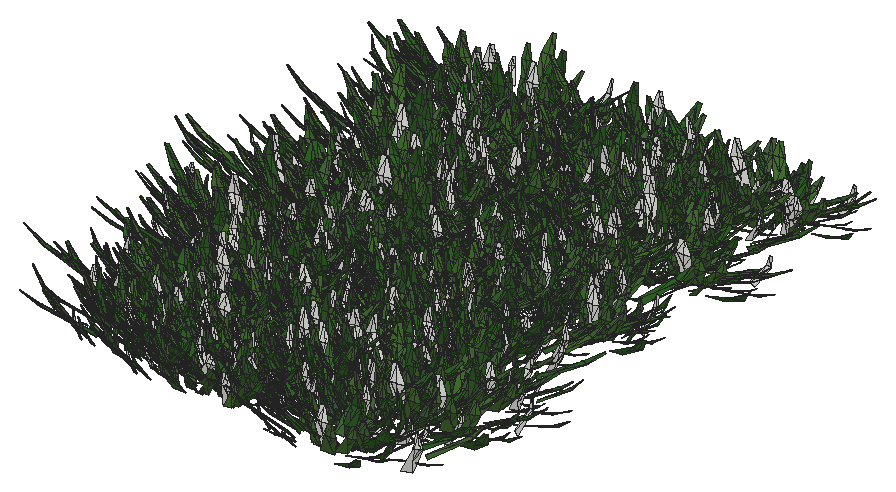
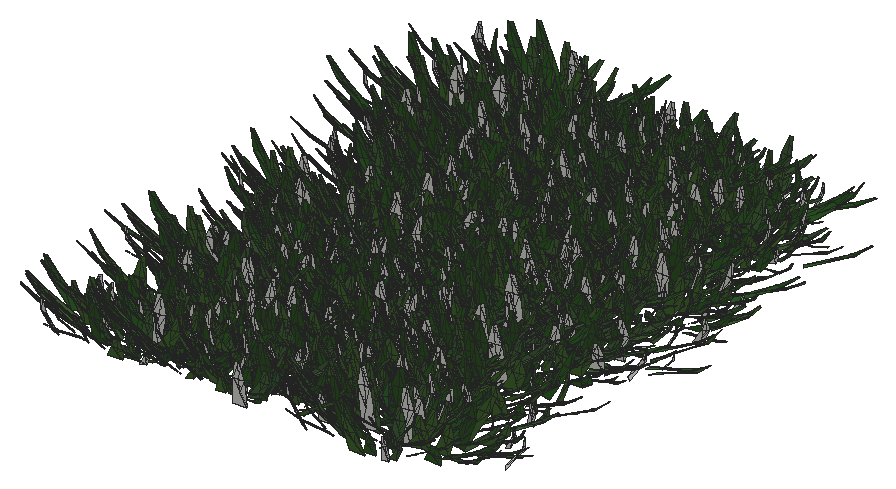
# SketchUp Ruby script. Lengths in inches.
U = 1.inch
M = Sketchup.active_model
def pt(a) = Geom::Point3d.new(a.map { |v| v * U })
def face(e, loops, mat)
  f = e.add_face(loops[0].map { |a| pt(a) })
  loops[1..].each { |l| e.add_face(l.map { |a| pt(a) }).erase! }
  f.material = f.back_material = mat if mat
  f
end
# faces: each face lists its corners as indices into pts; further lists are holes
def faces(e, pts, list, mat = nil) = list.each { |f| face(e, (f[0].is_a?(Array) ? f : [f]).map { |l| l.map { |i| pts[i] } }, mat) }
# xy, xz, yz: faces in a plane at the given z, y or x. An outline is a flat list of corners, or four numbers for a rectangle; further outlines are holes
def ring(l) = l.size == 4 ? [[l[0], l[1]], [l[2], l[1]], [l[2], l[3]], [l[0], l[3]]] : l.each_slice(2).to_a
def flat(e, list, mat, &to3) = list.each { |f| face(e, (f[0].is_a?(Array) ? f : [f]).map { |l| ring(l).map { |u, v| to3.(u, v) } }, mat) }
def xy(e, z, list, mat = nil) = flat(e, list, mat) { |x, y| [x, y, z] }
def xz(e, y, list, mat = nil) = flat(e, list, mat) { |x, z| [x, y, z] }
def yz(e, x, list, mat = nil) = flat(e, list, mat) { |y, z| [x, y, z] }
def lines(e, pts, list) = list.each { |a, b| e.add_line(pt(pts[a]), pt(pts[b])) }
# prism: a flat outline (further loops are holes) pulled along v
def prism(e, loops, v, mat = nil)
  f = face(e, loops, mat); d = Geom::Vector3d.new(v.map { |x| x * U })
  f.pushpull(f.normal.samedirection?(d) ? d.length : -d.length)
end
def box(e, o, s, mat = nil) = prism(e, [[o, [o[0] + s[0], o[1], o[2]], [o[0] + s[0], o[1] + s[1], o[2]], [o[0], o[1] + s[1], o[2]]]], [0, 0, s[2]], mat)
def at(x, y, z, deg = 0) = Geom::Transformation.translation(pt([x, y, z])) * Geom::Transformation.rotation(ORIGIN, Z_AXIS, deg.degrees)
def axes(o, x, y, z) = Geom::Transformation.new([*x, 0, *y, 0, *z, 0, *pt(o).to_a, 1])
def part(name) = M.definitions.add(name)
# library, detail: a bought-in or finely detailed component or shape, given as its bounding box
def library(name, o, s) = part(name).tap { |d| box(d.entities, o, s) }
def detail(e, o, s) = box(e.add_group.entities, o, s)
def put(e, d, t, mat = nil) = e.add_instance(d, t).tap { |i| i.material = mat if mat }
def group(e, t, mat = nil) = e.add_group.tap { |g| g.transformation = t; g.material = mat if mat }.entities
root = M.entities
M.materials.add("Material82").color = [68, 110, 58]
M.materials.add("Material83").color = [48, 90, 38]
M.materials.add("Material84").color = [68, 110, 48]
M.materials.add("Material85").color = [48, 90, 48]
M.materials.add("Material86").color = [58, 110, 58]
M.materials.add("Material87").color = [58, 90, 38]
M.materials.add("Material88").color = [68, 100, 58]
M.materials.add("Material89").color = [48, 100, 38]
c1 = part("grass00")
p = [[-0.6875,0.15,0],[-0.56,0.08,5.52],[-0.04,0.03,2.76],[0.48,-0.02,0],[0.35,-0.02,5.52],[-0.1,-0.14,5.52],
  [-0.12,0.65,8.37],[-0.42,0.65,8.37]]
faces(c1.entities,p,[[0,1,2,3],[3,2,4],[1,5,2],[5,4,2],[1,6,5],[4,5,6],[7,6,1]])
c2 = part("Group16\#1")
put(c2.entities,c1,axes([1.44,-0.61,-0.01],[0.05352,0.12609,0],[-0.10704,0.04543,0.07239],[0.06664,-0.02828,0.11628]),"Material85")
put(c2.entities,c1,axes([0.76,-0.15,-0.01],[0.04676,0.24062,0],[-0.23162,0.04501,0.06642],[0.0652,-0.01267,0.23595]),"Material82")
put(c2.entities,c1,axes([0.79,0.01,-0.01],[-0.00606,0.34651,0],[-0.34381,-0.00602,0.0432],[0.04319,0.00076,0.34386]))
put(c2.entities,c1,axes([1,0.23,-0.01],[-0.07192,0.31144,0],[-0.28722,-0.06632,0.1236],[0.12043,0.02781,0.29478]),"Material84")
put(c2.entities,c1,axes([1.66,0.77,-0.01],[-0.13828,0.29651,0],[-0.21551,-0.1005,0.22471],[0.20365,0.09498,0.23779]),"Material89")
put(c2.entities,c1,axes([0.6875,0.52,-0.01],[-0.18126,0.24051,0],[-0.22746,-0.17142,0.09788],[0.07817,0.05891,0.28481]),"Material84")
put(c2.entities,c1,axes([0.68,0.78,-0.01],[-0.215,0.18688,0],[-0.12385,-0.14248,0.21334],[0.13995,0.16101,0.18878]),"Material82")
put(c2.entities,c1,axes([0.56,1,-0.01],[-0.13756,0.07624,0],[-0.06159,-0.11112,0.0927],[0.04494,0.08108,0.12705]),"Material84")
put(c2.entities,c1,axes([0.2,0.64,-0.01],[-0.23729,0.07254,0],[-0.05711,-0.18681,0.153],[0.04473,0.14632,0.19535]),"Material89")
put(c2.entities,c1,axes([0.0625,0.72,-0.01],[-0.28874,0.02525,0],[-0.02179,-0.24916,0.14647],[0.01276,0.14591,0.25012]),"Material82")
put(c2.entities,c1,axes([-0.08,0.62,-0.01],[-0.34089,-0.04187,0],[0.03255,-0.26504,0.216],[-0.02633,0.21439,0.26703]),"Material89")
put(c2.entities,c1,axes([-0.34,0.98,-0.01],[-0.14314,-0.0493,0],[0.04397,-0.12769,0.06843],[-0.02228,0.0647,0.13505]),"Material89")
put(c2.entities,c1,axes([-0.87,1.45,-0.01],[-0.23488,-0.14114,0],[0.13761,-0.22901,0.06087],[-0.03135,0.05217,0.26717]))
put(c2.entities,c1,axes([-0.72,0.77,-0.01],[-0.14208,-0.13251,0],[0.07209,-0.0773,0.16301],[-0.11118,0.11922,0.1057]),"Material89")
put(c2.entities,c1,axes([-0.62,0.43,-0.01],[-0.14845,-0.21203,0],[0.18654,-0.13061,0.12304],[-0.10079,0.07057,0.22772]),"Material82")
put(c2.entities,c1,axes([-0.68,0.29,-0.01],[-0.13639,-0.32136,0],[0.31723,-0.13464,0.05579],[-0.05136,0.0218,0.34462]),"Material83")
put(c2.entities,c1,axes([-0.64,0.125,-0.01],[-0.0458,-0.23569,0],[0.22124,-0.043,0.08276],[-0.08124,0.01579,0.22538]),"Material86")
put(c2.entities,c1,axes([-1.6,-0.03,-0.01],[0.00576,-0.32897,0],[0.27526,0.00482,0.18018],[-0.18015,-0.00315,0.2753]),"Material84")
put(c2.entities,c1,axes([-1.36,-0.31,-0.01],[0.05718,-0.24765,0],[0.18172,0.04196,0.17267],[-0.16825,-0.03885,0.1865]),"Material89")
put(c2.entities,c1,axes([-1.54,-0.72,-0.01],[0.06537,-0.14017,0],[0.13555,0.06321,0.03939],[-0.0357,-0.01665,0.14956]))
put(c2.entities,c1,axes([-1.19,-0.9,-0.01],[0.09597,-0.12735,0],[0.11214,0.08451,0.07557],[-0.06035,-0.04548,0.14042]),"Material88")
put(c2.entities,c1,axes([-0.47,-0.54,-0.01],[0.11588,-0.10072,0],[0.0618,0.0711,0.12124],[-0.07953,-0.0915,0.0942]))
put(c2.entities,c1,axes([-0.47,-0.84,-0.01],[0.11927,-0.0661,0],[0.06603,0.11913,0.00646],[-0.00313,-0.00565,0.13621]),"Material84")
put(c2.entities,c1,axes([-0.38,-1.24,-0.01],[0.28037,-0.08571,0],[0.0618,0.20215,0.20315],[-0.05939,-0.19428,0.21139]),"Material88")
put(c2.entities,c1,axes([-0.06,-0.66,-0.01],[0.22719,-0.01987,0],[0.01247,0.14255,0.17758],[-0.01547,-0.17691,0.1431]),"Material87")
put(c2.entities,c1,axes([0.11,-0.89,-0.01],[0.14882,0.01828,0],[-0.01058,0.08611,0.12229],[0.01491,-0.12138,0.08676]),"Material85")
put(c2.entities,c1,axes([0.25,-0.72,-0.01],[0.20481,0.07053,0],[-0.06206,0.18022,0.10291],[0.03351,-0.0973,0.1906]),"Material85")
put(c2.entities,c1,axes([0.85,-1.42,-0.01],[0.16481,0.09904,0],[-0.09472,0.15762,0.05616],[0.02893,-0.04814,0.18389]),"Material84")
put(c2.entities,c1,axes([1.01,-1.09,-0.01],[0.21858,0.20385,0],[-0.17495,0.1876,0.15339],[0.10462,-0.11218,0.25652]),"Material89")
put(c2.entities,c1,axes([1.01,-0.71,-0.01],[0.08733,0.12473,0],[-0.06445,0.04512,0.13037],[0.1068,-0.07477,0.07867]),"Material85")
c3 = part("Group15\#1")
put(c3.entities,c2,at(0,0,0))
c4 = part("3darcstudiotree_grass00\#1")
put(c4.entities,c3,at(0,0,0))
put(root,c4,axes([650.38,940.35,-29.74],[0.55958,-1.81201,0],[3.80263,0.18264,-0.0324],[0.16574,0.00796,1.47946]))
put(root,c4,axes([635.88,940.68,-29.74],[3.74746,0.48768,0],[-1.05117,1.25627,-0.0401],[-0.08448,0.10096,1.69032]))
put(root,c4,axes([652.35,941.68,-29.74],[-3.98203,-0.87024,0],[2.1917,-1.55976,-0.02403],[0.066,-0.04697,1.92026]))
put(root,c4,axes([638.66,941.92,-29.74],[-3.4101,0.33219,0],[-0.86784,-1.38556,-0.03348],[-0.045,-0.07185,1.52035]))
put(root,c4,axes([627.54,942.55,-29.74],[3.16343,0.45899,0],[-1.51538,1.62437,-0.05896],[-0.12026,0.12891,1.94308]))
put(root,c4,axes([646.83,942.79,-29.74],[2.81615,0.69239,0],[-1.81737,1.14964,-0.0044],[-0.01183,0.00748,1.30779]))
put(root,c4,axes([634.52,943.04,-29.74],[3.17869,1.06939,0],[-2.97014,1.37309,-0.05603],[-0.1904,0.08802,1.79617]))
put(root,c4,axes([635.47,944.17,-29.74],[4.17705,-0.03481,0],[0.09875,1.84286,-0.00824],[0.00079,0.01483,1.59977]))
put(root,c4,axes([630.67,943.97,-29.74],[-4.39724,-0.41789,0],[0.97106,-1.58919,-0.03666],[0.03598,-0.05889,1.30149]))
put(root,c4,axes([646.32,945.17,-29.74],[3.16975,0.46707,0],[-1.43384,1.51339,-0.02415],[-0.05301,0.05595,1.92547]))
put(root,c4,axes([640.46,944.65,-29.74],[-0.72391,1.71321,0],[-3.27988,-0.21555,-0.00349],[-0.01869,-0.00123,1.35435]))
put(root,c4,axes([650.3,945.14,-29.74],[-2.94402,-0.61655,0],[1.96985,-1.46292,-0.05452],[0.11404,-0.08469,1.404]))
put(root,c4,axes([640.29,945.91,-29.74],[-3.95806,-0.26007,0],[0.56997,-1.34913,-0.01531],[0.01744,-0.04128,1.80136]))
put(root,c4,axes([635.75,946.01,-29.74],[-4.52935,0.02332,0],[-0.05756,-1.73901,-0.02897],[-0.00164,-0.04958,1.4344]))
put(root,c4,axes([652.69,946.56,-29.74],[-2.23453,-0.97852,0],[2.77364,-0.9851,-0.04825],[0.23755,-0.08437,1.85346]))
put(root,c4,axes([627.13,946.37,-29.74],[-3.49662,-0.83415,0],[2.45665,-1.60161,-0.00291],[0.00652,-0.00425,1.54121]))
put(root,c4,axes([646.06,946.48,-29.74],[-3.15856,-0.38514,0],[1.26271,-1.61061,-0.02785],[0.04659,-0.05943,1.81462]))
put(root,c4,axes([651.32,948.31,-29.74],[1.39356,-1.72752,0],[4.38256,0.54985,-0.00448],[0.02218,0.00278,1.79011]))
put(root,c4,axes([646.9375,948.29,-29.74],[3.28885,0.70173,0],[-2.10741,1.53616,-0.00222],[-0.00511,0.00372,1.6055]))
put(root,c4,axes([625.14,948.71,-29.74],[1.45525,-1.36358,0],[3.3603,0.55776,-0.00467],[0.02235,0.00371,1.41828]))
put(root,c4,axes([655.99,949.04,-29.74],[0.57397,-1.69302,0],[4.41794,0.23295,-0.0102],[0.05353,0.00282,1.76846]))
put(root,c4,axes([628.28,948.57,-29.74],[0.70399,1.48206,0],[-4.34932,0.32132,-0.00799],[-0.0357,0.00264,1.50733]))
put(root,c4,axes([633.28,949.06,-29.74],[0.05707,-1.33182,0],[4.67038,0.03113,-0.02351],[0.10833,0.00072,1.61343]))
put(root,c4,axes([640.61,949.375,-29.74],[2.93587,-1.18133,0],[2.75704,1.06566,-0.0131],[0.05816,0.02248,1.79861]))
put(root,c4,axes([640.14,950.18,-29.74],[0.93986,-1.61608,0],[3.43783,0.31095,-0.013],[0.09422,0.00852,1.96601]))
put(root,c4,axes([630.97,950.68,-29.74],[-3.07103,-1.30718,0],[3.25603,-1.18973,-0.02123],[0.06738,-0.02462,1.43939]))
put(root,c4,axes([624.84,950.39,-29.74],[-3.95181,0.01249,0],[-0.03447,-1.69649,-0.00779],[-0.00033,-0.01629,1.71052]))
put(root,c4,axes([634.71,950.92,-29.74],[-3.14814,-1.33954,0],[3.08708,-1.12839,-0.01903],[0.08494,-0.03105,1.91973]))
put(root,c4,axes([649.76,950.75,-29.74],[-3.70599,0.79197,0],[-2.20745,-1.60656,-0.0133],[-0.03552,-0.02585,1.94738]))
put(root,c4,axes([645.39,951.125,-29.74],[-1.513,1.21159,0],[-3.36011,-0.6526,-0.03193],[-0.17356,-0.03371,1.70102]))
put(root,c4,axes([651.1,952.375,-29.74],[-0.43315,-1.7077,0],[3.80872,-0.15025,-0.05423],[0.31945,-0.0126,1.69842]))
put(root,c4,axes([629.79,953.12,-29.74],[3.9873,-0.15062,0],[0.35569,1.46445,-0.02913],[0.01977,0.08141,1.9903]))
put(root,c4,axes([645.58,953.14,-29.74],[3.21716,0.40848,0],[-1.16198,1.42335,-0.048],[-0.09517,0.11657,1.83855]))
put(root,c4,axes([640.55,953.36,-29.74],[-0.9687,-1.6973,0],[3.99206,-0.35436,-0.03143],[0.1527,-0.01355,1.52743]))
put(root,c4,axes([655.0625,953.78,-29.74],[2.35188,-1.38482,0],[3.12769,0.82614,-0.05113],[0.23612,0.06237,1.56833]))
put(root,c4,axes([635.875,953.33,-29.74],[-2.94959,0.77761,0],[-1.85667,-1.09533,-0.00767],[-0.02785,-0.01643,1.63569]))
put(root,c4,axes([640.42,954.69,-29.74],[-0.43954,-1.59759,0],[3.53501,-0.15126,-0.05057],[0.33495,-0.01433,1.77563]))
put(root,c4,axes([627.3,955.23,-29.74],[0.98995,-1.43102,0],[4.03348,0.43397,-0.01691],[0.08344,0.00898,1.6028]))
put(root,c4,axes([647.4375,955.49,-29.74],[3.3322,0.38036,0],[-1.11394,1.51777,-0.02015],[-0.03056,0.04163,1.63787]))
put(root,c4,axes([654.87,955.36,-29.74],[-3.1964,-0.45712,0],[1.21547,-1.32188,-0.00444],[0.00788,-0.00857,1.39182]))
put(root,c4,axes([634.13,955.57,-29.74],[-1.72626,1.58438,0],[-3.31687,-0.56206,-0.02574],[-0.1159,-0.01964,1.32606]))
put(root,c4,axes([651.18,956.01,-29.74],[-3.35036,0.87409,0],[-2.07562,-1.23735,-0.03289],[-0.10016,-0.05971,1.55622]))
put(root,c4,axes([632.68,956.9,-29.74],[2.55829,-1.10547,0],[3.21956,1.15881,-0.03913],[0.13719,0.04938,1.55084]))
put(root,c4,axes([651.21,957.42,-29.74],[4.04553,0.2871,0],[-0.83462,1.82911,-0.01866],[-0.01606,0.0352,1.717]))
put(root,c4,axes([624.46,957.74,-29.74],[2.65299,-0.97546,0],[3.20943,1.35758,-0.02398],[0.06395,0.02705,1.37951]))
put(root,c4,axes([646.53,957.51,-29.74],[-3.75328,0.12847,0],[-0.28677,-1.30306,-0.03872],[-0.02406,-0.10934,1.78675]))
put(root,c4,axes([629.3,957.78,-29.74],[-3.24632,0.41503,0],[-1.13877,-1.38534,-0.02033],[-0.04358,-0.05301,1.92362]))
put(root,c4,axes([639.89,958.09,-29.74],[-3.60435,-0.22712,0],[0.60496,-1.49319,-0.01241],[0.00897,-0.02215,1.31731]))
put(root,c4,axes([641.47,958.9375,-29.74],[1.97331,-1.7001,0],[3.41411,0.61633,-0.04178],[0.21918,0.03957,1.62381]))
put(root,c4,axes([628.76,959.1,-29.74],[-1.21684,1.60263,0],[-3.24686,-0.38342,-0.04102],[-0.25836,-0.03051,1.67021]))
put(root,c4,axes([625.61,959.22,-29.74],[-4.06047,-0.30244,0],[0.85134,-1.77769,-0.03943],[0.03436,-0.07175,1.61444]))
put(root,c4,axes([643.84,959.59,-29.74],[3.0128,0.96923,0],[-2.26467,1.09486,-0.0073],[-0.03331,0.01611,1.93831]))
put(root,c4,axes([649.92,959.93,-29.74],[-2.43541,-1.16543,0],[2.64027,-0.85812,-0.03867],[0.17422,-0.05662,1.49724]))
put(root,c4,axes([632.875,960.5,-29.74],[-3.18803,-0.40221,0],[1.38309,-1.70502,-0.00535],[0.00805,-0.00992,1.67969]))
put(root,c4,axes([651.92,961.28,-29.74],[-2.79186,-1.03231,0],[2.26214,-0.95152,-0.04465],[0.21173,-0.08906,1.71883]))
put(root,c4,axes([624.28,961.18,-29.74],[-1.54224,1.54277,0],[-3.96225,-0.61604,-0.03242],[-0.18554,-0.02885,1.96368]))
put(root,c4,axes([633.7,961.25,-29.74],[-2.16052,1.42464,0],[-3.02099,-0.71254,-0.01081],[-0.04852,-0.01144,1.38013]))
put(root,c4,axes([639.64,961.87,-29.74],[3.59479,1.11581,0],[-2.65109,1.32837,-0.01986],[-0.0739,0.03703,1.93312]))
put(root,c4,axes([629.01,962.29,-29.74],[4.36912,-0.54802,0],[1.07763,1.33621,-0.00335],[0.00554,0.00687,1.45436]))
put(root,c4,axes([646.16,962.06,-29.74],[0.73987,1.59354,0],[-4.44696,0.32112,-0.04305],[-0.22862,0.01651,1.82947]))
put(root,c4,axes([622.9375,963.26,-29.74],[3.29517,0.70525,0],[-2.24642,1.63243,-0.00178],[-0.00323,0.00235,1.34491]))
put(root,c4,axes([650.43,963.76,-29.74],[-3.56566,-0.8896,0],[2.32838,-1.45148,-0.01513],[0.04457,-0.02778,1.79885]))
put(root,c4,axes([629.49,963.88,-29.74],[1.39223,1.25256,0],[-3.795,0.65605,-0.01361],[-0.06427,0.01111,1.60179]))
put(root,c4,axes([633.26,964.22,-29.74],[1.97793,1.10174,0],[-3.47293,0.96971,-0.06047],[-0.20758,0.05796,1.34144]))
put(root,c4,axes([643.89,964.26,-29.74],[-2.92804,-0.86099,0],[2.52273,-1.33432,-0.01853],[0.05328,-0.02818,1.52144]))
put(root,c4,axes([639.22,964.65,-29.74],[-1.63823,-1.36099,0],[3.49292,-0.65391,-0.00409],[0.01763,-0.0033,1.3842]))
put(root,c4,axes([639.09,965.68,-29.74],[2.36777,-1.25491,0],[3.70344,1.08678,-0.00846],[0.02737,0.00803,1.39582]))
put(root,c4,axes([651.37,965.51,-29.74],[-3.34111,0.18713,0],[-0.56421,-1.56678,-0.00819],[-0.00515,-0.01431,1.3463]))
put(root,c4,axes([646.61,965.92,-29.74],[0.58066,1.77085,0],[-3.90665,0.19923,-0.04685],[-0.26361,0.01344,1.67517]))
put(root,c4,axes([633.67,966.68,-29.74],[-4.52964,-0.09494,0],[0.22898,-1.69903,-0.02618],[0.00745,-0.05528,1.73378]))
put(root,c4,axes([628.67,966.96,-29.74],[-2.17136,1.02025,0],[-2.89421,-0.95801,-0.02769],[-0.1122,-0.03714,1.49833]))
put(root,c4,axes([639.4,968.42,-29.74],[3.08639,0.66231,0],[-1.76537,1.27948,-0.04213],[-0.09869,0.07153,1.35679]))
put(root,c4,axes([655.41,968.78,-29.74],[1.1756,-1.47793,0],[3.44657,0.42639,-0.02865],[0.17647,0.02183,1.74795]))
put(root,c4,axes([624.96,968.89,-29.74],[4.53982,0.21063,0],[-0.49544,1.66085,-0.02625],[-0.01899,0.06364,1.96735]))
put(root,c4,axes([633.02,969.01,-29.74],[0.12157,-1.62148,0],[4.39568,0.05126,-0.0158],[0.08264,0.00096,1.72451]))
put(root,c4,axes([647.74,968.9,-29.74],[-1.04498,-1.27032,0],[4.0983,-0.52433,-0.01227],[0.0665,-0.00851,1.83962]))
put(root,c4,axes([652.89,968.89,-29.74],[2.22198,1.23467,0],[-3.2898,0.92081,-0.0048],[-0.02055,0.00575,1.58899]))
put(root,c4,axes([627.65,969.1875,-29.74],[3.78243,-0.20016,0],[0.50434,1.48226,-0.04419],[0.03105,0.09126,1.50171]))
put(root,c4,axes([646.57,969.88,-29.74],[3.7109,-0.91214,0],[2.11846,1.34044,-0.04378],[0.13838,0.08756,1.79394]))
put(root,c4,axes([638.78,970.45,-29.74],[3.96894,-0.58875,0],[1.33194,1.3965,-0.01237],[0.02838,0.02976,1.84855]))
put(root,c4,axes([631.15,970.52,-29.74],[0.11291,-1.83708,0],[4.52912,0.0433,-0.04883],[0.22915,0.00219,1.59403]))
put(root,c4,axes([624.1,970.91,-29.74],[4.70379,-0.18713,0],[0.44198,1.72795,-0.01121],[0.00446,0.01743,1.30781]))
put(root,c4,axes([636.02,971.21,-29.74],[2.20471,-1.56419,0],[3.09714,0.67895,-0.02727],[0.12975,0.02844,1.44583]))
put(root,c4,axes([650.26,971.18,-29.74],[2.778,0.72584,0],[-2.53603,1.50959,-0.00365],[-0.00789,0.0047,1.34685]))
put(root,c4,axes([646.26,972.25,-29.74],[3.34228,0.13265,0],[-0.43082,1.68835,-0.00091],[-0.00041,0.00162,1.45853]))
put(root,c4,axes([651.98,972.03,-29.74],[3.42042,0.9713,0],[-2.12433,1.16348,-0.02682],[-0.10129,0.05548,1.76121]))
put(root,c4,axes([640.62,972.11,-29.74],[3.30561,0.92504,0],[-2.54174,1.41264,-0.05586],[-0.15004,0.08339,1.52805]))
put(root,c4,axes([634.125,973.27,-29.74],[2.97087,-0.63768,0],[1.76888,1.28171,-0.04084],[0.13668,0.09904,1.94165]))
put(root,c4,axes([629.25,973.18,-29.74],[-4.25587,0.04591,0],[-0.1089,-1.57017,-0.04984],[-0.00682,-0.0984,1.49526]))
put(root,c4,axes([629.22,974.41,-29.74],[0.66389,-1.49509,0],[4.57403,0.31589,-0.04237],[0.23153,0.01599,1.93074]))
put(root,c4,axes([623.625,974.33,-29.74],[-0.08871,1.46443,0],[-4.0853,-0.03849,-0.0357],[-0.16722,-0.00158,1.43525]))
put(root,c4,axes([633.36,974.75,-29.74],[-4.65824,0.34825,0],[-0.74927,-1.55877,-0.04366],[-0.04609,-0.09588,1.70895]))
put(root,c4,axes([640.85,975.62,-29.74],[-1.5733,-1.53629,0],[3.8056,-0.60614,-0.01424],[0.06159,-0.00981,1.43479]))
put(root,c4,axes([651.4,975.46,-29.74],[-3.34476,-0.15722,0],[0.48645,-1.60959,-0.01308],[0.00826,-0.02735,1.64432]))
put(root,c4,axes([644.1875,975.79,-29.74],[-3.6982,-1.11774,0],[2.6803,-1.37926,-0.01589],[0.04062,-0.0209,1.38765]))
put(root,c4,axes([629.51,977.21,-29.74],[3.97153,-0.13343,0],[0.30373,1.40602,-0.01096],[0.00672,0.03109,1.93666]))
put(root,c4,axes([645.85,977.11,-29.74],[1.27309,1.64144,0],[-4.4392,0.53549,-0.03143],[-0.12353,0.0149,1.42994]))
put(root,c4,axes([635.75,977.33,-29.74],[-2.73035,-0.81396,0],[2.55013,-1.33042,-0.03674],[0.11326,-0.05909,1.62045]))
put(root,c4,axes([649.66,977.35,-29.74],[-0.26231,1.84263,0],[-3.30675,-0.07321,-0.00552],[-0.03272,-0.00072,1.47331]))
put(root,c4,axes([638.26,977.54,-29.74],[-4.55367,0.27818,0],[-0.67765,-1.72528,-0.03016],[-0.02264,-0.05764,1.62739]))
put(root,c4,axes([627.39,978.96,-29.74],[2.00913,-1.08398,0],[3.65765,1.05439,-0.0361],[0.15471,0.0446,1.80295]))
put(root,c4,axes([647.8,979.02,-29.74],[1.02841,-1.31305,0],[3.38391,0.41221,-0.03395],[0.18437,0.02246,1.50895]))
put(root,c4,axes([641.46,978.55,-29.74],[-3.47148,-0.32447,0],[1.09042,-1.81447,-0.00987],[0.00954,-0.01587,1.48448]))
put(root,c4,axes([651.53,979.17,-29.74],[3.21897,1.19921,0],[-3.23164,1.34914,-0.01632],[-0.04651,0.01942,1.46423]))
put(root,c4,axes([633.1,979.78,-29.74],[3.35413,-0.63199,0],[1.61191,1.33051,-0.01719],[0.04506,0.03719,1.70421]))
put(root,c4,axes([649.3,980.94,-29.74],[3.19452,-0.59612,0],[1.46474,1.2208,-0.01286],[0.03129,0.02608,1.45976]))
put(root,c4,axes([642.14,981.03,-29.74],[4.44722,-0.53115,0],[1.26492,1.64719,-0.03542],[0.04521,0.05887,1.44036]))
put(root,c4,axes([655.6,981.01,-29.74],[0.90068,-1.41561,0],[4.53027,0.44829,-0.03647],[0.13709,0.01357,1.35653]))
put(root,c4,axes([630.27,981.27,-29.74],[4.35154,-0.63119,0],[1.42423,1.52711,-0.01984],[0.04228,0.04533,1.90869]))
put(root,c4,axes([643.86,981.38,-29.74],[-4.1478,0.13224,0],[-0.279,-1.36104,-0.02584],[-0.01399,-0.06822,1.74304]))
put(root,c4,axes([636.18,982.21,-29.74],[1.55533,-1.52655,0],[4.26431,0.67573,-0.03894],[0.20513,0.0325,1.95573]))
put(root,c4,axes([624.11,982.24,-29.74],[1.46562,-1.72266,0],[4.03529,0.53396,-0.04434],[0.25483,0.03372,1.93394]))
put(root,c4,axes([630.81,983.45,-29.74],[0.94741,-1.42267,0],[3.73003,0.38633,-0.03356],[0.18091,0.01874,1.61101]))
put(root,c4,axes([646.83,983.51,-29.74],[3.53019,1.19751,0],[-2.61374,1.19838,-0.04839],[-0.15514,0.07113,1.47711]))
put(root,c4,axes([651.97,983.24,-29.74],[-2.66899,1.32243,0],[-3.00544,-0.94339,-0.02078],[-0.10429,-0.03273,1.84714]))
put(root,c4,axes([632.78,984.29,-29.74],[3.44825,-0.26897,0],[0.66516,1.32629,-0.00259],[0.00332,0.00662,1.70099]))
put(root,c4,axes([641.59,984.23,-29.74],[1.7248,1.72946,0],[-3.94677,0.61218,-0.01805],[-0.10059,0.0156,1.90362]))
put(root,c4,axes([651.08,985.43,-29.74],[4.2125,0.29861,0],[-0.756,1.65872,-0.00017],[-0.00017,0.00037,1.78268]))
put(root,c4,axes([628.4,985.46,-29.74],[3.77678,0.27869,0],[-0.6902,1.45473,-0.00485],[-0.00557,0.01174,1.75633]))
put(root,c4,axes([647.29,986,-29.74],[1.40396,-1.3283,0],[3.66211,0.60201,-0.02113],[0.09939,0.01634,1.51549]))
put(root,c4,axes([634.02,985.83,-29.74],[-3.60203,-0.72226,0],[1.64221,-1.27378,-0.05096],[0.13667,-0.10601,1.60728]))
put(root,c4,axes([642.29,986.68,-29.74],[2.99585,-0.78884,0],[2.43675,1.4393,-0.03164],[0.10153,0.05997,1.90074]))
put(root,c4,axes([624.6,987.37,-29.74],[3.00061,-1.20381,0],[2.59687,1.00673,-0.02297],[0.10061,0.039,1.67632]))
put(root,c4,axes([630.68,987.7,-29.74],[2.81234,1.34734,0],[-2.81254,0.91306,-0.01155],[-0.05543,0.018,1.69697]))
put(root,c4,axes([641.55,988.21,-29.74],[3.0975,-0.44176,0],[1.39811,1.52468,-0.04794],[0.07202,0.07854,1.36124]))
put(root,c4,axes([643.75,988.2,-29.74],[2.38875,-0.89777,0],[2.38741,0.98797,-0.03437],[0.15253,0.06312,1.66865]))
put(root,c4,axes([651.5,987.84,-29.74],[-4.04939,0.05434,0],[-0.15117,-1.75202,-0.01213],[-0.00231,-0.02678,1.86653]))
put(root,c4,axes([635,988.4375,-29.74],[-1.19412,-1.34448,0],[3.1862,-0.44013,-0.02961],[0.14836,-0.02049,1.34337]))
put(root,c4,axes([650.3125,989.65,-29.74],[-2.58541,-0.85496,0],[2.80483,-1.31917,-0.0116],[0.03194,-0.01502,1.40225]))
put(root,c4,axes([628.7,989.56,-29.74],[-3.45253,0.27622,0],[-0.72182,-1.40321,-0.01756],[-0.02267,-0.04407,1.76676]))
put(root,c4,axes([646.97,990.17,-29.74],[0.99609,-1.23763,0],[4.45512,0.55768,-0.04397],[0.17141,0.02146,1.43296]))
put(root,c4,axes([639.89,989.76,-29.74],[-4.42879,-0.33071,0],[0.76141,-1.58586,-0.02653],[0.02727,-0.05679,1.69452]))
put(root,c4,axes([634.39,990.76,-29.74],[-3.59651,-0.44623,0],[1.25179,-1.56915,-0.00258],[0.00335,-0.0042,1.35273]))
put(root,c4,axes([634.6,991.78,-29.74],[3.47707,-0.28838,0],[0.88445,1.65855,-0.04208],[0.03591,0.06734,1.3356]))
put(root,c4,axes([623.41,991.65,-29.74],[0.85595,1.34318,0],[-4.39323,0.43542,-0.04255],[-0.19043,0.01887,1.5668]))
put(root,c4,axes([644.45,992.3125,-29.74],[0.38467,-1.72776,0],[3.7527,0.12994,-0.02351],[0.1369,0.00474,1.65028]))
put(root,c4,axes([640.71,991.85,-29.74],[-3.45853,-0.30921,0],[0.875,-1.52216,-0.03754],[0.05438,-0.09459,1.94323]))
put(root,c4,axes([653.22,992.52,-29.74],[-1.62678,1.3546,0],[-3.70168,-0.6914,-0.05633],[-0.31213,-0.0583,1.88219]))
put(root,c4,axes([627.23,992.54,-29.74],[-2.26736,0.9467,0],[-3.26135,-1.21483,-0.01576],[-0.0639,-0.0238,1.87507]))
put(root,c4,axes([641.93,994.12,-29.74],[4.2542,-0.55295,0],[1.2277,1.46904,-0.0158],[0.03318,0.0397,1.97161]))
put(root,c4,axes([628.7,994.43,-29.74],[0.78455,-1.57227,0],[3.87046,0.30038,-0.05061],[0.32766,0.02543,1.95081]))
put(root,c4,axes([645.8125,993.85,-29.74],[-4.20928,0.13814,0],[-0.29813,-1.41294,-0.01346],[-0.00713,-0.03379,1.72106]))
put(root,c4,axes([655.49,994.56,-29.74],[1.41685,-1.43454,0],[3.76136,0.57778,-0.0174],[0.0698,0.01072,1.30214]))
put(root,c4,axes([652,993.97,-29.74],[-3.91283,-0.66077,0],[1.78522,-1.64415,-0.00601],[0.01088,-0.01002,1.5624]))
